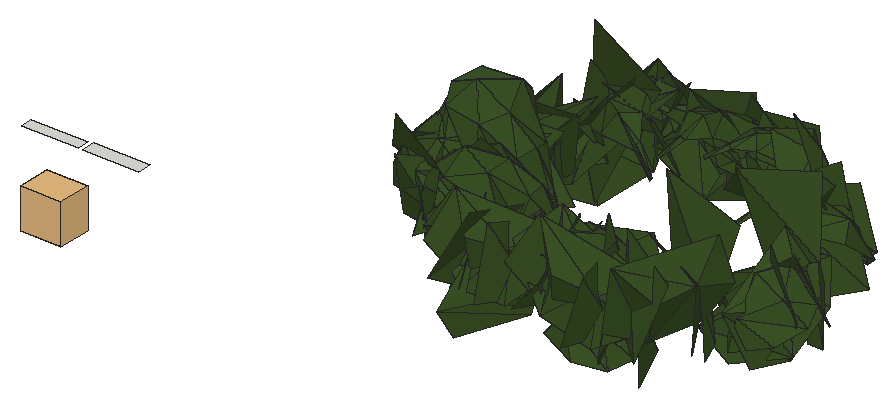
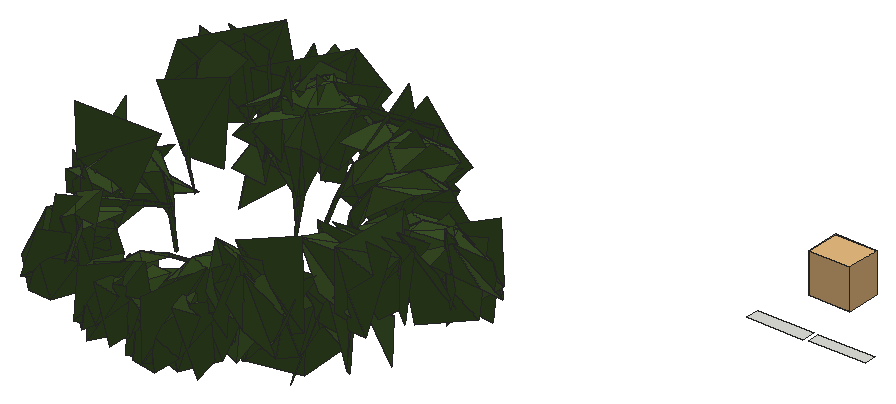
# SketchUp Ruby script. Lengths in inches.
U = 1.inch
M = Sketchup.active_model
def pt(a) = Geom::Point3d.new(a.map { |v| v * U })
def face(e, loops, mat)
  f = e.add_face(loops[0].map { |a| pt(a) })
  loops[1..].each { |l| e.add_face(l.map { |a| pt(a) }).erase! }
  f.material = f.back_material = mat if mat
  f
end
# faces: each face lists its corners as indices into pts; further lists are holes
def faces(e, pts, list, mat = nil) = list.each { |f| face(e, (f[0].is_a?(Array) ? f : [f]).map { |l| l.map { |i| pts[i] } }, mat) }
# xy, xz, yz: faces in a plane at the given z, y or x. An outline is a flat list of corners, or four numbers for a rectangle; further outlines are holes
def ring(l) = l.size == 4 ? [[l[0], l[1]], [l[2], l[1]], [l[2], l[3]], [l[0], l[3]]] : l.each_slice(2).to_a
def flat(e, list, mat, &to3) = list.each { |f| face(e, (f[0].is_a?(Array) ? f : [f]).map { |l| ring(l).map { |u, v| to3.(u, v) } }, mat) }
def xy(e, z, list, mat = nil) = flat(e, list, mat) { |x, y| [x, y, z] }
def xz(e, y, list, mat = nil) = flat(e, list, mat) { |x, z| [x, y, z] }
def yz(e, x, list, mat = nil) = flat(e, list, mat) { |y, z| [x, y, z] }
def lines(e, pts, list) = list.each { |a, b| e.add_line(pt(pts[a]), pt(pts[b])) }
# prism: a flat outline (further loops are holes) pulled along v
def prism(e, loops, v, mat = nil)
  f = face(e, loops, mat); d = Geom::Vector3d.new(v.map { |x| x * U })
  f.pushpull(f.normal.samedirection?(d) ? d.length : -d.length)
end
def box(e, o, s, mat = nil) = prism(e, [[o, [o[0] + s[0], o[1], o[2]], [o[0] + s[0], o[1] + s[1], o[2]], [o[0], o[1] + s[1], o[2]]]], [0, 0, s[2]], mat)
def at(x, y, z, deg = 0) = Geom::Transformation.translation(pt([x, y, z])) * Geom::Transformation.rotation(ORIGIN, Z_AXIS, deg.degrees)
def axes(o, x, y, z) = Geom::Transformation.new([*x, 0, *y, 0, *z, 0, *pt(o).to_a, 1])
def part(name) = M.definitions.add(name)
# library, detail: a bought-in or finely detailed component or shape, given as its bounding box
def library(name, o, s) = part(name).tap { |d| box(d.entities, o, s) }
def detail(e, o, s) = box(e.add_group.entities, o, s)
def put(e, d, t, mat = nil) = e.add_instance(d, t).tap { |i| i.material = mat if mat }
def group(e, t, mat = nil) = e.add_group.tap { |g| g.transformation = t; g.material = mat if mat }.entities
root = M.entities
M.materials.add("AM113_062_Tilia").color = [58, 81, 37]
c1 = library("Plante \#58",[-0.43,-1.58,0],[20.84,18.06,17.59])
xy(root,469.24,[[748.74,187.1875,835.24,205.25],[841.77,187.1875,927.68,207.4375]])
p = [[1701.59,327.72,485.11],[1747.62,323.99,427.11],[1744.9375,404.02,402.97],[1744.625,377.27,484.06],[1733.1,431.27,507.89],[1738.64,469.02,442.6],
  [1768.29,437.47,411.79],[1735.83,448.95,403.14],[1695,492.42,498.26],[1265.87,545.37,425.47],[1282.25,519.69,404.47],[1322.11,458.22,479.16],
  [1336,548.89,407.3125],[1307.39,502.99,433.22],[1309.27,556.05,487.21],[1366.9,616.33,435.07],[1642.86,241.01,515.23],[1650.1,233.87,408.15],
  [1621.58,305.75,416.66],[1665.8125,616.23,495.33],[1638.09,510.87,529.97],[1716.79,588.29,408.72],[1676.24,514.1,412.62],[1276.875,506.84,503.81],
  [1249.57,481.03,409.31],[1293.41,422.13,436.62],[1430.65,632.1,410.51],[1368.87,622.77,454.14],[1399.73,657.93,507.43],[1448.28,674.23,474.2],
  [1507.55,658.02,499.97],[1501.79,670.07,419.95],[1363.54,272.6,524.11],[1339.37,262.72,421.625],[1400.99,309.14,410.57],[1386.73,383.1,479.77],
  [1513.04,600.03,501.53],[1515.51,652.04,439.02],[1437.35,653.31,411.2],[1460.93,652.04,491.83],[1370.28,650.18,448.97],[1407.47,648.14,513.43],
  [1706.97,493.33,528.125],[1769.35,437.02,502.12],[1312.18,567.02,412.06],[1293.01,516.33,434.07],[1321.22,552.28,496.57],[1350.48,631.13,447.7],
  [1373.7,273.49,413.75],[1421.08,270.06,444.32],[1379.66,304.51,484.51],[1307.16,305.73,424.43],[1543.88,299.5,480.84],[1614.57,433.17,416.67],
  [1636.86,411.59,454.4],[1633.03,416.9,457.83],[1611.57,434.61,420.04],[1653.71,341.92,444.18],[1720.79,318.13,428.22],[1759.09,390.59,417.67],
  [1715.5,373.74,481.14],[1720.33,427.53,504.78],[1761.92,458.19,457.59],[1634.98,422.08,454.28],[1615.25,435.74,418.21],[1400.53,161.25,455.3],
  [1414.93,175.95,418.67],[1480.5,241.4,444.88],[1254.1,347.73,419.15],[1272.51,301.42,445.67],[1235.46,334.9375,495.54],[1222.25,409.9375,442.37],
  [1280.27,573.11,523.38],[1304.11,604.75,419.85],[1344.52,532.18,421.76],[1689.81,620.6875,420.04],[1678.61,616.42,468.17],[1701.28,571.09,507.91],
  [1719.86,595.78,447.95],[1654.27,623.01,420.78],[1580.64,586.3,455.8],[1621.89,607.43,477.04],[1521.5,598.08,522.81],[1518.34,620.33,425.31],
  [1557.5625,675.3,421.59],[1548.48,683.15,511.8125],[1399.4375,531.38,527.97],[1330.2,330.06,500.55],[1318.44,404.14,506.86],[1266.33,355.77,490.37],
  [1227.25,340.57,425.16],[1254.48,298.38,447.4],[1245.25,341.98,503.43],[1202.24,406.65,455.22],[1699.57,624.3125,438.28],[1686.63,593.3,425.31],
  [1606.45,569.38,482.9],[1321.95,462.18,511.88],[1293.57,542.3,506.82],[1413.56,693.26,524.91],[1390.14,674.3,426.08],[1370.89,610.65,474.66],
  [1578.3125,635.85,504.09],[1581.43,647.58,439.53],[1516.38,651.19,428.5],[1544.625,672.3,482.25],[1468.45,670.14,461.87],[1503.23,680.97,507.26],
  [1557.79,593.26,503.24],[1582.91,629.07,454.65],[1529.9,663.1,430.07],[1543.65,651.37,496.01],[1504.35,670.85,511.95],[1481.05,688.64,458.78],
  [1492.74,661.44,486.05],[1507.82,642.03,453.34],[1474.63,691.23,431.26],[1432.25,702.7,433.65],[1207.17,324.48,531.23],[1194.86,356.3125,432.75],
  [1271.66,345.07,432.13],[1305.85,389.16,527.26],[1720.78,291.15,466.21],[1698.92,298.95,432.3],[1638.4,369.03,458.78],[1446.1,709.58,443.64],
  [1440.6,676.57,432.66],[1410.17,624.25,524.38],[1630.32,182,460.16],[1612.79,204.03,433.17],[1599.54,289.92,482.17],[1315.29,493.67,506.9],
  [1444.75,694.33,479.49],[1404.53,691.4,457.21],[1350.71,480.32,473.03],[1506.1875,339.2,434.33],[1506.9,324.61,485.99],[1509.55,331.12,485.06],
  [1670.67,374.55,438.11],[1709.21,329.75,434.33],[1715.1,339.82,478.09],[1768.07,343.61,455.93],[1506.17,343.32,435.5625],[1514.29,330.71,479.96],
  [1508.87,340.32,434.62],[1325.01,613.13,512.26],[1365.63,626.42,584.18],[1366.19,674.45,520.33],[1395.35,396.47,468.94],[1404,420.97,435.25],
  [1405.13,424,438.52],[1401.7,422.71,435.79],[1385.95,397.56,475.27],[1392.9375,398.52,475.79],[1375.86,455.82,460.99],[1659.06,384.47,470.35],
  [1597.01,584.3,507.66],[1666.96,634.51,517.15],[1527.19,699.49,523.18],[1505.53,697.32,441.6875],[1464.25,660.64,478.09],[1202.625,379.94,517.38],
  [1217.47,420.18,581.47],[1180.7,445.55,521.55],[1724.375,493.65,501.66],[1561.71,201.25,493.5625],[1596.48,172.92,450.7],[1636.56,191.62,442.99],
  [1620.52,205.63,485.42],[1649.84,224.28,449.4375],[1511.18,331.66,443.21],[1529.9,303.33,476.46],[1530.74,310.05,479.09],[1510.72,334.74,446.91],
  [1533.61,312.99,473.12],[1513.47,333.46,443.34],[1408.39,634.11,554.875],[1450.22,706.11,532.32],[1671.39,483.61,497.6875],[1444.04,335.07,455.9],
  [1412.47,549.6,551.67],[1407.75,614.97,444.81],[1335.55,667.01,466.3],[1485.04,248.39,476.76],[1285.59,304.67,513.89],[1314.82,322.0625,479.86],
  [1348.87,599.3125,531.9],[1422.0625,598.58,574.97],[1386.46,662.65,543.21],[1718.41,542.54,490.71],[1300.27,410.02,548.31],[1246.66,439.75,448.54],
  [1167.58,416.67,473.4],[1558.72,698.11,458.79],[1541.34,677.63,448.45],[1495.93,653,519.97],[1569.83,644.61,492.54],[1573.01,625.18,465.67],
  [1571.15,673.54,448.8],[1546.48,699.26,450.06],[1346.35,645.86,508.65],[1628.48,262.36,495.71],[1631.25,307.34,470.29],[1423.4,299.2,550.35],
  [1402.38,242.58,449.65],[1383.1875,167.25,492.71],[1603.53,538.66,536.27],[1616.34,578.6,450.13],[1672.65,613.94,465.91],[1550.47,687.67,487.22],
  [1521.89,702.78,467.98],[1537.86,194,460.3],[1491.96,312.31,504.57],[1524.06,228.85,450.67],[1541.4375,178.08,535.04],[1748.74,407.4,545.74],
  [1719.6,472.47,450.95],[1648.59,414.34,465.68],[1784.33,429.67,452.45],[1786.28,365.56,483.85],[1766.96,381.12,451.87],[1695.98,433.64,496.55],
  [1297.62,490.31,452.6],[1297.2,419.35,457.15],[1272.8,434.05,528.78],[1264.45,490.76,528.08],[1294.02,532.5,579],[1275.63,555.96,506.74],
  [1478.06,599.84,488.12],[1345.24,628.52,515],[1242.34,445.63,559.34],[1249.32,455.17,454.24],[1310.83,412.5,474.03],[1662.63,402.24,496.8125],
  [1677.16,425.66,498.88],[1362.22,480.75,569.22],[1332.41,506.07,454.48],[1252.33,526.57,467.63],[1376.34,291.88,499.76],[1414.65,300.73,461.64],
  [1393.73,341.02,455.05],[1394.1875,344.99,492.58],[1226.86,390.46,534.09],[1269.92,445.81,569.02],[1201.47,454.6875,541.52],[1416.64,207.5,519.88],
  [1603.35,547.99,468.87],[1789.7,380.43,472.64],[1295.03,268.74,488.71],[1306.31,291.17,457.11],[1392.3,326.89,480.33],[1290.97,378.75,500.52],
  [1373.9,630.04,522.65],[1407.66,664.71,520.05],[1740.36,486.38,508.51],[1587.24,299.42,458.24],[1582.09,294.26,494.93],[1637.69,379.35,489.66],
  [1498.04,660.24,545.03],[1557.83,692.93,530.66],[1461.09,694.98,506.36],[1270.39,426.32,459.125],[1273.85,384.39,499.13],[1284.32,437.5,536.15],
  [1278.33,499.12,461.3],[1376.11,406.47,504.9375],[1383.03,415.24,459.65],[1386.93,416.42,460.36],[1606.89,294.84,513.8125],[1623.16,212.6,540.89],
  [1383.06,418.13,460.15],[1374.04,414.43,513.69],[1378.83,409.77,510.7],[1531.93,252.85,462.21],[1289.86,492.88,545.81],[1351.8,528.43,570.87],
  [1297.29,559.15,527.23],[1337.77,260.86,464.61],[1452.89,683.34,510.8],[1419.33,209,462.09],[1417.15,194.44,548.15],[1372.31,233.43,584.12],
  [1474.4375,204.84,548.08],[1351.45,197.86,520.23],[1491.17,212.33,469.81],[1289.84,604.9,462.15],[1319.21,517.02,466.8125],[1304.7,557.32,506.3125],
  [1303.56,618.49,518.4],[1297.82,641.13,473.46],[1538.64,269.34,492.22],[1422.61,361.93,528.54],[1347.32,323.44,462.88],[1290.56,302.63,539.22],
  [1456.77,349.49,463.17],[1437.6,347.88,512.25],[1444.34,345.73,512.37],[1460.73,349.82,465.02],[1548.77,196.87,480.83],[1618.09,211.75,463.5],
  [1621.56,191.74,540.95],[1665.97,218.4,494.3],[1444.75,340.95,507.33],[1458.05,346.9,463.68],[1671.25,554.99,531.68],[1683.49,576.82,473.625],
  [1625.26,606.32,463.96],[1654.7,604.32,523.2],[1617.34,622.59,550.1],[1584.83,634.58,502.46],[1302.55,265.08,468.79],[1319.23,284.625,506.95],
  [1533.76,607.97,491.43],[1659.77,606.875,555.46],[1688.05,319.55,537.18],[1303.44,599.37,541.83],[1364.04,532.38,482.35],[1251.9,479.02,562.29],
  [1473.22,672.27,517.83],[1511.25,682.2,517.97],[1643.38,585.21,511.35],[1404.36,583.6,572.18],[1337.66,592.29,468.25],[1263.82,628.85,514.84],
  [1301.47,340.32,519.9],[1276.1,298.95,484.33],[1380.24,364.68,509.875],[1607.08,557.43,504.42],[1687.04,440.83,469.06],[1730.38,422.25,522.16],
  [1712.99,466.25,504.79],[1637.08,524.68,515.92],[1677.0625,556.79,481.74],[1641.93,611.65,469.68],[1645.24,583.3,529.15],[1614.4,612.22,551.1],
  [1603.37,647.0625,506],[1531.03,217.9375,516.0625],[1546.2,176.89,494.03],[1617.93,184.0625,470.26],[1616.79,203.1,548.125],[1664.27,200.21,496.37],
  [1704.7,391.03,515.21],[1759.21,374.27,503.4],[1779.57,412.23,488.7],[1558.84,283.27,507.875],[1187.62,347.39,473.22],[1269.58,319.375,476.0625],
  [1232.36,332.97,513.67],[1186.62,367.33,524.61],[1165.54,374.29,482.95],[1201.27,357.23,546.6],[1357.44,627,560.28],[1330.5625,662.47,508.875],
  [1296.66,647.57,496.19],[1326.56,633.15,473.59],[1342.81,535.25,501.13],[1358.05,456.14,557.17],[1445.64,581.66,530.29],[1359.16,380.38,500.04],
  [1283.97,361.85,487.24],[1336.55,382.26,476.13],[1282.53,361.125,491.2],[1622.59,162.32,577.63],[1594.17,156.78,476.43],[1624.35,228.29,476.65],
  [1585.16,273.96,567.22],[1410.58,192.01,477.65],[1484.71,186.54,481.86],[1470.39,217.6,550.58],[1375.23,287.68,553.9],[1346.95,223.52,531.5],
  [1413.74,223.14,555.34],[1502.56,608.46,524.05],[1445.24,652.42,529.06],[1579.79,265.03,606.23],[1603.73,215.9375,524.55],[1601.77,285.39,479.93],
  [1517.37,320.34,498.49],[1520.13,314.25,536.79],[1547.4375,313.91,531.66],[1404.52,321.39,509.1875],[1480.125,246.6,577.125],[1494.22,189.47,543.22],
  [1553.625,219.12,480.61],[1543.99,234.4,565.6],[1584.625,275.37,555.53],[1608.4,266.1,480.68],[1629.08,307.875,515.61],[1530.04,197.05,618.59],
  [1499.6,166.85,556.53],[1568.67,171.58,558.5625],[1658.59,169.85,601.05],[1661.85,148.77,522.6],[1671.94,223.71,480.89],[1703.5625,199.06,552.24],
  [1723.14,253.32,562.48],[1706.28,286.09,495.96],[1160.625,377.93,504.2],[1187.77,391.04,481.07],[1270.23,348.45,506.26],[1462.43,182,589.06],
  [1456.15,163.89,484.06],[1497.19,229.73,481.16],[1448.87,293.27,541.39],[1745.78,225.23,587.43],[1732.01,232.2,481.41],[1697.82,296.6,515.71],
  [1525.8,200.8,521.13],[1612.83,465.96,592.6],[1661.69,463.73,482.02],[1743.22,461.48,511.01],[1356.86,529.59,521.66],[1211.84,413.58,559.76],
  [1169.1,411.96,513.5],[1700.41,362.72,590.32],[1592.62,360.43,630.39],[1679.68,337.51,483.78],[1599.87,361.09,503.42],[1691.06,434.04,529.58],
  [1743.75,368.5625,555.53],[1562.47,274.125,586.24],[1525.77,228.0625,484.07],[1526.83,146.15,511.31],[1721.375,199.67,586.68],[1621.89,248.89,607.9],
  [1695.64,168.55,484.64],[1633.3,225.73,485.01],[1689.96,464.46,541.26],[1591.31,251.09,511.73],[1499.86,300.39,521.2],[1469.61,601.21,523.65],
  [1282.88,356.39,524.43],[1531.96,657.78,525.79],[1336.47,284.4375,558.67],[1664.86,518.4,499.92],[1527.5625,612.06,520.0625],[1359.1,324.96,521.03],
  [1428.22,190.7,586.71],[1519.16,254.04,603.59],[1494.9,189.57,575.52],[1563.6875,197.94,574.14],[1662.37,232.98,561.98],[1732.45,314.26,544.72],
  [1327.12,522.06,525.57],[1285.68,598.11,567.46],[1654.79,265.07,526.3],[1322.45,393.98,520.89],[1349.45,410.75,496.85],[1352,411.24,500.95],
  [1349.01,413.41,498.28],[1315.94,400.07,528.44],[1321.44,395.63,528.47],[1606.9375,503.19,513.07],[1596.52,469.6,498.92],[1595.95,468.02,503.75],
  [1414.63,520.45,522.22],[1447.58,508.53,498.89],[1449.45,506.67,503.42],[1336.23,385.48,535.5],[1610.18,503.73,519.84],[1598.97,468.23,499.95],
  [1616.97,504.41,517.47],[1644.875,528.36,524.375],[1379.5,628.29,568.39],[1301.79,391.3,566.46],[1415,522.34,530.39],[1449.47,510.63,500.59],
  [1415.19,529.9,530.43],[1560.75,302.97,500.98],[1577.96,278.24,571.76],[1601.1,305.7,528.39],[1371.48,589.87,547.79],[1493.54,276.13,501.63],
  [1478.45,224.65,533.82],[1496.39,239.02,569.34],[1571.15,642.7,554.11],[1454.07,645.1,536.58],[1475.2,668.17,554.99],[1271.67,330.24,530.26],
  [1192.71,344.3125,571.79],[1624,545.8125,528.23],[1547.89,250.29,601.23],[1363.8125,397.99,562.95],[1352.15,374.25,552.76],[1583.27,650.93,553.92],
  [1333.66,568.83,545.72],[1486.74,639.5,506.6],[1500.14,639.88,531.45],[1423.64,334.12,561.35],[1425.8,306.84,556.7],[1408.76,603.7,508.93],
  [1423.25,613.5,538.63],[1389.2,644.6,544.22],[1497.99,596.02,527.37],[1478.16,572.62,514.37],[1479.34,573.32,510.38],[1502.28,596.62,522.7],
  [1720.01,495.3,612.63],[1493.85,597.04,524.15],[1477.55,574.68,511.18],[1588.65,165.05,589.86],[1409.86,353.23,543.38],[1216.4375,446.51,542.38],
  [1241.16,362.4,548.28],[1357.91,424.01,555.07],[1292.85,597.96,623.72],[1592.21,335.14,553.78],[1637.03,270.21,598.91],[1556.55,603.07,565.59],
  [1448.85,565.75,535.05],[1442.54,528,521.03],[1443.24,529.35,516.03],[1452.87,568.94,529],[1515.78,243.33,575.19],[1443.75,564.07,531.32],
  [1440.51,529.68,517.08],[1387.18,357.625,520.14],[1332.12,368.93,543.97],[1344.4,352.27,581.75],[1516.52,625.72,536.86],[1285.02,375.57,549.89],
  [1521.85,269.71,532.02],[1537.39,282.27,572.79],[1373.26,540.13,550.28],[1311.05,353.29,594.38],[1322.99,329.29,541.18],[1334.1875,371.28,523.04],
  [1449.67,609.19,544.64],[1389.04,273.88,591.625],[1421.95,252.7,553.18],[1418.78,292.62,524.8125],[1592.43,223.97,563.75],[1282.43,402.8,548.85],
  [1356.42,301.88,616.07],[1270.64,425.01,529.45],[1394.72,560.0625,550.96],[1406.84,584.62,531.27],[1582.92,612.3,591.46],[1525.79,191.66,565.61],
  [1255.19,361.61,596.89],[1307.7,442,617.28],[1336.65,441.91,543.15],[1298.65,469.36,589.73],[1389.9375,314.65,592.52],[1300.03,319.38,571.35],
  [1718.62,300.51,610.47],[1330.99,388.33,602.26],[1337.12,255.35,575.66],[1570.07,196.55,569.02],[1552.63,228.01,589.08],[1307.83,275.61,576.3],
  [1335.84,295.44,600.69],[1252.55,433.56,619.38],[1276.98,391.97,628.21],[1239.63,391.13,612.95]]
faces(root,p,[[0,1,2],[2,3,0],[4,3,2],[2,5,4],[6,7,8],[9,10,11],[12,13,14],[15,12,14],
  [16,17,18],[19,20,21],[20,22,21],[23,24,25],[26,27,28],[28,29,26],[30,31,26],[26,29,30],
  [32,33,34],[32,34,35],[36,37,38],[38,39,36],[38,40,41],[41,39,38],[42,43,6],[8,42,6],
  [44,45,46],[47,44,46],[48,49,50],[51,48,50],[16,18,52],[53,54,55],[55,56,53],[57,58,59],
  [59,60,57],[61,60,59],[59,62,61],[63,64,56],[65,66,67],[68,69,70],[71,68,70],[72,73,74],
  [56,55,63],[75,76,77],[77,78,75],[75,79,76],[79,80,81],[76,79,81],[82,83,84],[85,82,84],
  [72,74,86],[50,87,51],[88,89,51],[51,87,88],[90,91,92],[93,90,92],[94,95,96],[11,97,9],
  [97,98,9],[99,100,101],[102,103,104],[104,105,102],[104,106,107],[107,105,104],[108,109,110],[110,111,108],
  [112,111,110],[110,113,112],[114,115,116],[114,116,117],[118,119,120],[118,120,121],[122,123,124],[125,126,127],
  [128,129,130],[14,13,131],[117,132,114],[117,133,132],[46,45,134],[135,136,137],[138,139,140],[140,139,141],
  [137,142,135],[143,144,142],[14,145,15],[15,145,146],[146,147,15],[148,149,150],[142,137,143],[151,152,153],
  [153,150,151],[23,25,154],[140,155,138],[96,156,94],[156,157,94],[150,153,148],[158,159,160],[70,161,71],
  [71,161,162],[162,163,71],[5,164,4],[165,166,167],[167,168,165],[167,169,168],[170,171,172],[172,173,170],
  [174,175,173],[127,176,125],[176,177,125],[61,178,57],[57,60,61],[50,49,179],[180,181,182],[67,183,65],
  [70,69,184],[173,172,174],[92,91,185],[46,186,47],[47,186,187],[187,188,47],[77,189,78],[190,191,192],
  [193,194,195],[196,197,198],[196,198,199],[40,200,41],[168,169,201],[169,202,201],[203,204,205],[206,207,208],
  [199,209,196],[199,210,209],[165,211,166],[212,213,214],[215,216,217],[215,218,216],[219,220,221],[222,223,224],
  [224,225,222],[222,225,226],[226,227,222],[228,115,114],[27,229,28],[230,231,232],[63,55,233],[233,234,63],
  [54,155,233],[233,55,54],[235,236,237],[238,239,240],[240,241,238],[92,242,93],[93,242,243],[243,244,93],
  [183,245,65],[81,80,246],[50,179,88],[140,141,247],[248,249,250],[223,251,224],[133,252,253],[132,133,253],
  [62,254,61],[255,256,201],[201,202,255],[124,257,122],[195,258,193],[258,259,193],[113,260,112],[261,262,263],
  [264,261,263],[265,266,267],[130,268,128],[268,269,128],[270,271,272],[272,267,270],[273,211,165],[267,272,265],
  [263,274,264],[264,274,275],[275,276,264],[277,239,238],[106,278,107],[279,280,281],[282,280,279],[281,283,279],
  [279,284,282],[285,286,287],[288,285,287],[289,285,288],[165,290,273],[291,292,293],[294,295,296],[296,297,294],
  [298,299,300],[299,301,300],[302,303,297],[304,305,306],[306,307,304],[308,307,306],[306,309,308],[310,277,311],
  [311,277,238],[297,296,302],[312,197,196],[313,206,208],[257,314,122],[315,180,182],[287,286,316],[317,235,237],
  [210,318,319],[209,210,319],[77,76,320],[321,322,323],[320,76,81],[324,325,310],[310,311,324],[326,241,148],
  [148,153,326],[246,327,81],[328,234,329],[329,330,328],[331,332,333],[333,334,331],[335,334,333],[333,336,335],
  [284,337,282],[338,339,340],[339,341,340],[155,140,342],[342,233,155],[247,343,140],[247,344,343],[46,134,187],
  [174,172,345],[345,256,174],[346,347,348],[349,346,348],[350,346,349],[351,190,192],[289,288,352],[352,353,289],
  [354,355,356],[230,232,357],[30,29,28],[99,101,358],[152,359,326],[326,153,152],[348,347,360],[361,362,324],
  [324,359,361],[363,364,365],[171,290,345],[345,172,171],[363,365,366],[320,81,327],[367,368,369],[370,371,367],
  [367,372,370],[369,372,367],[140,343,342],[158,160,373],[374,132,253],[114,132,374],[375,376,377],[375,377,378],
  [92,185,243],[379,380,143],[143,137,379],[250,381,248],[382,383,384],[384,385,382],[386,385,384],[384,387,386],
  [387,388,386],[389,390,298],[298,391,389],[300,391,298],[392,393,394],[394,395,392],[396,395,394],[394,397,396],
  [398,399,400],[401,402,403],[401,403,404],[405,406,407],[368,408,369],[409,410,411],[102,105,107],[316,412,287],
  [350,349,413],[413,414,350],[415,416,417],[416,418,417],[221,419,219],[419,420,219],[421,422,423],[0,3,4],
  [324,362,325],[88,87,50],[424,425,426],[425,427,426],[379,137,136],[4,428,0],[165,168,429],[429,168,201],
  [136,430,379],[114,431,228],[431,114,374],[360,432,348],[14,131,146],[146,145,14],[196,209,433],[433,209,319],
  [381,434,248],[343,344,329],[344,330,329],[435,189,77],[196,436,312],[36,39,41],[290,165,429],[429,345,290],
  [436,196,433],[437,238,241],[437,241,326],[438,203,205],[439,440,338],[338,441,439],[340,441,338],[300,301,442],
  [429,256,345],[429,201,256],[70,184,162],[162,161,70],[397,443,396],[108,111,112],[444,445,354],[356,444,354],
  [340,341,446],[187,186,46],[342,234,233],[447,448,449],[61,254,178],[450,451,452],[452,449,450],[342,329,234],
  [453,454,455],[456,457,458],[263,262,459],[437,311,238],[460,455,461],[461,462,460],[77,463,435],[359,324,437],
  [437,326,359],[28,464,30],[224,251,465],[466,458,467],[467,468,466],[449,452,447],[469,380,470],[470,471,469],
  [41,472,36],[473,474,475],[475,430,473],[4,164,428],[309,476,308],[112,477,108],[243,242,92],[342,343,329],
  [458,466,456],[455,460,453],[107,478,102],[400,479,398],[479,480,398],[481,327,453],[320,327,481],[482,212,214],
  [483,484,265],[265,272,483],[336,485,335],[486,287,412],[486,288,287],[112,260,477],[319,318,487],[487,488,319],
  [324,311,437],[489,490,302],[302,296,489],[107,278,478],[28,229,464],[463,77,320],[41,200,472],[253,252,491],
  [491,492,253],[352,493,353],[494,495,496],[496,497,494],[483,272,271],[498,409,411],[499,500,495],[501,421,423],
  [320,481,463],[295,502,489],[489,296,295],[453,460,481],[413,503,414],[504,349,348],[504,348,432],[271,505,483],
  [495,494,499],[506,321,323],[386,388,507],[405,407,508],[335,509,331],[331,334,335],[510,511,512],[512,513,510],
  [282,337,514],[515,516,511],[481,460,462],[462,463,481],[433,319,488],[352,288,486],[374,253,492],[517,518,519],
  [519,502,517],[497,436,520],[433,520,436],[521,432,447],[447,452,521],[511,510,515],[369,408,522],[430,475,523],
  [523,379,430],[524,412,456],[486,412,524],[456,466,524],[520,494,497],[525,526,527],[527,484,525],[304,307,308],
  [513,431,528],[374,528,431],[499,494,520],[520,488,499],[504,432,521],[413,349,504],[529,530,531],[531,490,529],
  [433,488,520],[340,446,439],[226,225,224],[532,471,470],[451,533,521],[521,452,451],[534,291,293],[224,465,226],
  [528,510,513],[374,492,528],[413,533,535],[535,503,413],[524,466,468],[468,536,524],[352,536,537],[528,492,515],
  [515,510,528],[537,493,352],[523,470,380],[523,380,379],[308,538,304],[369,522,370],[475,474,539],[263,459,275],
  [275,274,263],[389,391,300],[300,442,389],[540,526,525],[541,505,542],[542,543,541],[502,519,544],[544,489,502],
  [519,518,545],[396,443,546],[486,524,536],[536,352,486],[281,280,282],[439,441,340],[282,514,281],[533,413,504],
  [504,521,533],[308,476,538],[370,372,369],[335,485,509],[392,395,396],[547,525,484],[547,484,483],[548,530,529],
  [386,507,382],[505,541,547],[547,483,505],[382,385,386],[544,529,490],[544,490,489],[396,546,392],[549,532,550],
  [550,532,470],[475,539,549],[549,550,475],[475,550,523],[519,545,551],[523,550,470],[551,548,552],[552,548,529],
  [551,552,519],[519,552,544],[541,543,553],[544,552,529],[554,540,525],[547,554,525],[555,540,554],[541,554,547],
  [541,553,555],[555,554,541]],"AM113_062_Tilia")
put(root,c1,axes([874.84,32.98,439.71],[2.9928,0,0],[0,2.7666,0],[0,0,3.48]))
